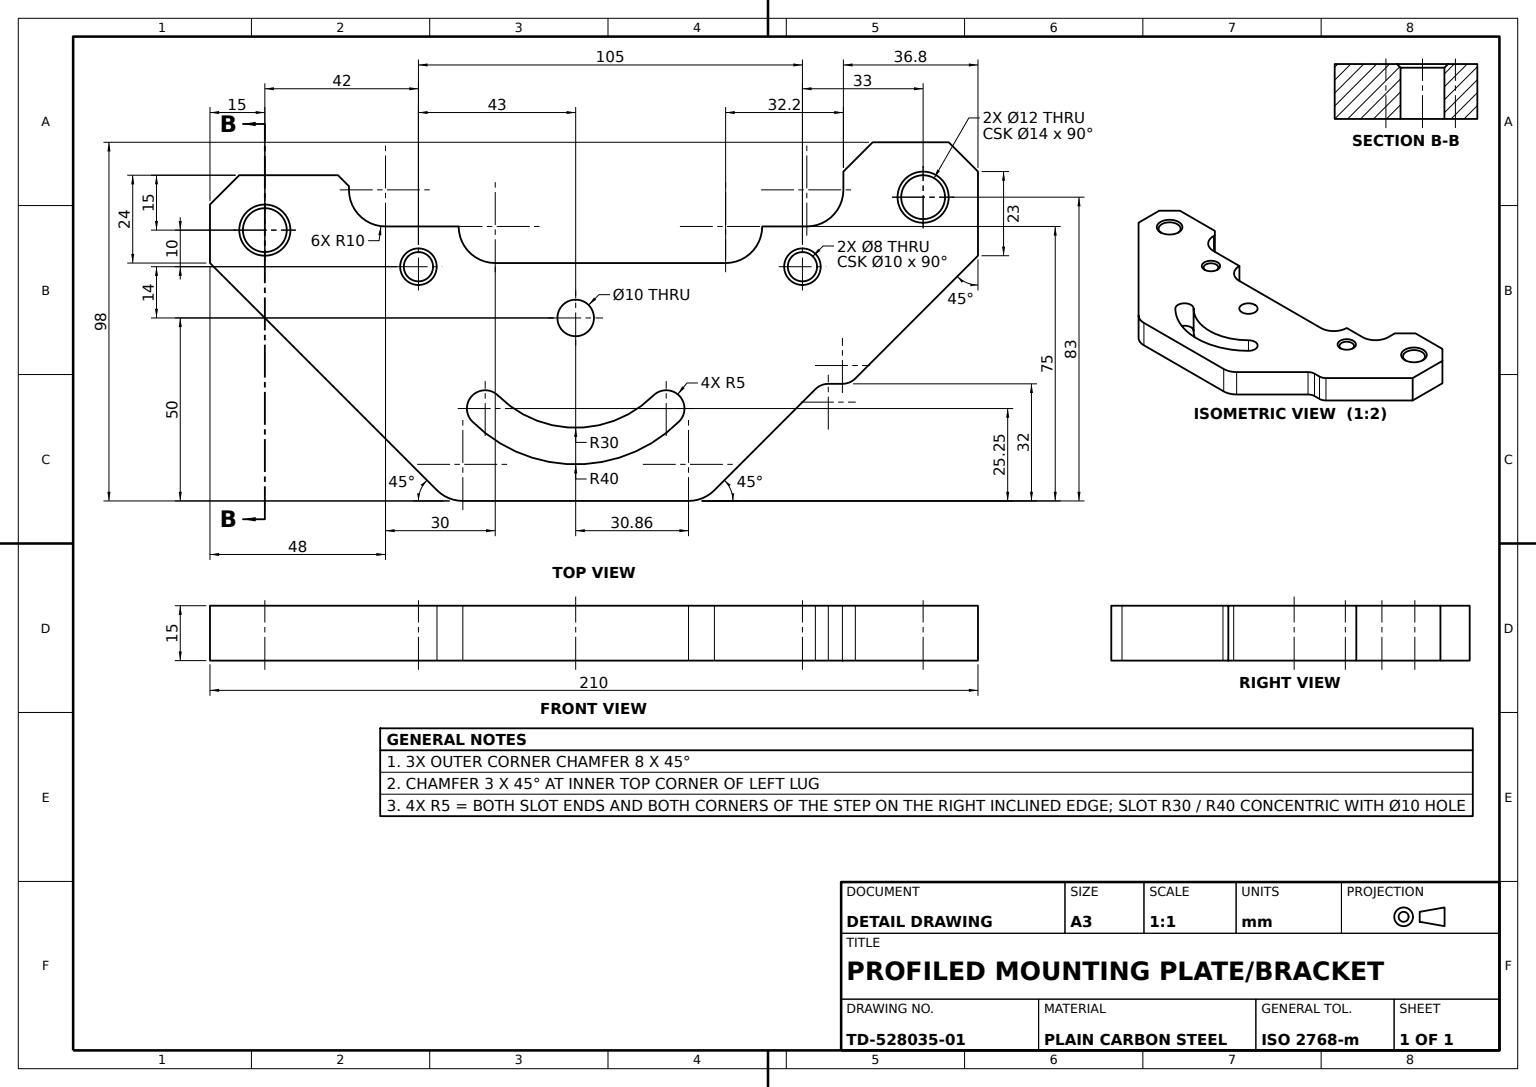
ISO-10303-21;
HEADER;
FILE_DESCRIPTION((''),'2;1');
FILE_NAME('','',(''),(''),'','','');
FILE_SCHEMA(('AUTOMOTIVE_DESIGN'));
ENDSEC;
DATA;
#1=APPLICATION_CONTEXT('');
#2=PRODUCT_CONTEXT('',#1,'mechanical');
#3=PRODUCT('','','',(#2));
#4=PRODUCT_DEFINITION_FORMATION('','',#3);
#5=PRODUCT_DEFINITION_CONTEXT('',#1,'design');
#6=PRODUCT_DEFINITION('','',#4,#5);
#7=PRODUCT_DEFINITION_SHAPE('','',#6);
#8=(LENGTH_UNIT()NAMED_UNIT(*)SI_UNIT(.MILLI.,.METRE.));
#9=(NAMED_UNIT(*)PLANE_ANGLE_UNIT()SI_UNIT($,.RADIAN.));
#10=(NAMED_UNIT(*)SI_UNIT($,.STERADIAN.)SOLID_ANGLE_UNIT());
#11=UNCERTAINTY_MEASURE_WITH_UNIT(LENGTH_MEASURE(1.E-05),#8,'distance_accuracy_value','');
#12=(GEOMETRIC_REPRESENTATION_CONTEXT(3)GLOBAL_UNCERTAINTY_ASSIGNED_CONTEXT((#11))GLOBAL_UNIT_ASSIGNED_CONTEXT((#8,#9,#10))REPRESENTATION_CONTEXT('',''));
#13=CARTESIAN_POINT('',(102.,15.,-48.));
#14=VERTEX_POINT('',#13);
#15=CARTESIAN_POINT('',(102.,0.,-48.));
#16=VERTEX_POINT('',#15);
#17=DIRECTION('',(0.,-1.,0.));
#18=VECTOR('',#17,1000.);
#19=LINE('',#13,#18);
#20=EDGE_CURVE('',#14,#16,#19,.T.);
#21=ORIENTED_EDGE('',*,*,#20,.F.);
#22=CARTESIAN_POINT('',(110.,15.,-40.));
#23=VERTEX_POINT('',#22);
#24=CARTESIAN_POINT('',(75.,15.,-75.));
#25=DIRECTION('',(-0.707106781,0.,-0.707106781));
#26=VECTOR('',#25,1000.);
#27=LINE('',#24,#26);
#28=EDGE_CURVE('',#23,#14,#27,.T.);
#29=ORIENTED_EDGE('',*,*,#28,.F.);
#30=CARTESIAN_POINT('',(110.,0.,-40.));
#31=VERTEX_POINT('',#30);
#32=DIRECTION('',(0.,1.,0.));
#33=VECTOR('',#32,1000.);
#34=LINE('',#22,#33);
#35=EDGE_CURVE('',#31,#23,#34,.T.);
#36=ORIENTED_EDGE('',*,*,#35,.F.);
#37=DIRECTION('',(0.707106781,0.,0.707106781));
#38=VECTOR('',#37,1000.);
#39=LINE('',#15,#38);
#40=EDGE_CURVE('',#16,#31,#39,.T.);
#41=ORIENTED_EDGE('',*,*,#40,.F.);
#42=EDGE_LOOP('',(#21,#29,#36,#41));
#43=FACE_OUTER_BOUND('',#42,.T.);
#44=DIRECTION('',(-0.707106781,0.,0.707106781));
#45=AXIS2_PLACEMENT_3D('',#13,#44,#17);
#46=PLANE('',#45);
#47=ADVANCED_FACE('',(#43),#46,.F.);
#48=CARTESIAN_POINT('',(-92.,0.,-39.));
#49=VERTEX_POINT('',#48);
#50=CARTESIAN_POINT('',(-65.,0.,-39.));
#51=VERTEX_POINT('',#50);
#52=CARTESIAN_POINT('',(0.,0.,-39.));
#53=DIRECTION('',(1.,0.,0.));
#54=VECTOR('',#53,1000.);
#55=LINE('',#52,#54);
#56=EDGE_CURVE('',#49,#51,#55,.T.);
#57=ORIENTED_EDGE('',*,*,#56,.F.);
#58=CARTESIAN_POINT('',(-92.,15.,-39.));
#59=VERTEX_POINT('',#58);
#60=LINE('',#58,#33);
#61=EDGE_CURVE('',#49,#59,#60,.T.);
#62=ORIENTED_EDGE('',*,*,#61,.T.);
#63=CARTESIAN_POINT('',(-65.,15.,-39.));
#64=VERTEX_POINT('',#63);
#65=CARTESIAN_POINT('',(0.,15.,-39.));
#66=LINE('',#65,#54);
#67=EDGE_CURVE('',#59,#64,#66,.T.);
#68=ORIENTED_EDGE('',*,*,#67,.T.);
#69=LINE('',#63,#18);
#70=EDGE_CURVE('',#64,#51,#69,.T.);
#71=ORIENTED_EDGE('',*,*,#70,.T.);
#72=EDGE_LOOP('',(#57,#62,#68,#71));
#73=FACE_OUTER_BOUND('',#72,.T.);
#74=DIRECTION('',(0.,0.,-1.));
#75=DIRECTION('',(-1.,0.,0.));
#76=AXIS2_PLACEMENT_3D('',#65,#74,#75);
#77=PLANE('',#76);
#78=ADVANCED_FACE('',(#73),#77,.T.);
#79=CARTESIAN_POINT('',(95.,14.,-39.));
#80=VERTEX_POINT('',#79);
#81=CARTESIAN_POINT('',(95.,14.,-27.));
#82=VERTEX_POINT('',#81);
#83=CARTESIAN_POINT('',(95.,14.,-33.));
#84=DIRECTION('',(0.,0.,1.));
#85=AXIS2_PLACEMENT_3D('',#83,#32,#84);
#86=CIRCLE('',#85,6.);
#87=EDGE_CURVE('',#80,#82,#86,.T.);
#88=ORIENTED_EDGE('',*,*,#87,.F.);
#89=CARTESIAN_POINT('',(95.,15.,-40.));
#90=VERTEX_POINT('',#89);
#91=DIRECTION('',(0.,0.707106781,-0.707106781));
#92=VECTOR('',#91,1000.);
#93=LINE('',#79,#92);
#94=EDGE_CURVE('',#80,#90,#93,.T.);
#95=ORIENTED_EDGE('',*,*,#94,.T.);
#96=CARTESIAN_POINT('',(95.,15.,-26.));
#97=VERTEX_POINT('',#96);
#98=CARTESIAN_POINT('',(95.,15.,-33.));
#99=AXIS2_PLACEMENT_3D('',#98,#17,#84);
#100=CIRCLE('',#99,7.);
#101=EDGE_CURVE('',#97,#90,#100,.T.);
#102=ORIENTED_EDGE('',*,*,#101,.F.);
#103=DIRECTION('',(0.,0.707106781,0.707106781));
#104=VECTOR('',#103,1000.);
#105=LINE('',#81,#104);
#106=EDGE_CURVE('',#82,#97,#105,.T.);
#107=ORIENTED_EDGE('',*,*,#106,.F.);
#108=EDGE_LOOP('',(#88,#95,#102,#107));
#109=FACE_OUTER_BOUND('',#108,.T.);
#110=CONICAL_SURFACE('',#85,6.,0.785398163);
#111=ADVANCED_FACE('',(#109),#110,.F.);
#112=CARTESIAN_POINT('',(-32.,15.,-25.));
#113=VERTEX_POINT('',#112);
#114=CARTESIAN_POINT('',(-32.,0.,-25.));
#115=VERTEX_POINT('',#114);
#116=LINE('',#112,#18);
#117=EDGE_CURVE('',#113,#115,#116,.T.);
#118=ORIENTED_EDGE('',*,*,#117,.F.);
#119=CARTESIAN_POINT('',(-22.,15.,-15.));
#120=VERTEX_POINT('',#119);
#121=CARTESIAN_POINT('',(-22.,15.,-25.));
#122=AXIS2_PLACEMENT_3D('',#121,#17,#84);
#123=CIRCLE('',#122,10.);
#124=EDGE_CURVE('',#120,#113,#123,.T.);
#125=ORIENTED_EDGE('',*,*,#124,.F.);
#126=CARTESIAN_POINT('',(-22.,0.,-15.));
#127=VERTEX_POINT('',#126);
#128=LINE('',#119,#33);
#129=EDGE_CURVE('',#127,#120,#128,.T.);
#130=ORIENTED_EDGE('',*,*,#129,.F.);
#131=CARTESIAN_POINT('',(-22.,0.,-25.));
#132=AXIS2_PLACEMENT_3D('',#131,#32,#84);
#133=CIRCLE('',#132,10.);
#134=EDGE_CURVE('',#115,#127,#133,.T.);
#135=ORIENTED_EDGE('',*,*,#134,.F.);
#136=EDGE_LOOP('',(#118,#125,#130,#135));
#137=FACE_OUTER_BOUND('',#136,.T.);
#138=AXIS2_PLACEMENT_3D('',#121,#32,#84);
#139=CYLINDRICAL_SURFACE('',#138,10.);
#140=ADVANCED_FACE('',(#137),#139,.F.);
#141=CARTESIAN_POINT('',(37.928932,15.,47.071068));
#142=VERTEX_POINT('',#141);
#143=CARTESIAN_POINT('',(37.928932,0.,47.071068));
#144=VERTEX_POINT('',#143);
#145=LINE('',#141,#18);
#146=EDGE_CURVE('',#142,#144,#145,.T.);
#147=ORIENTED_EDGE('',*,*,#146,.F.);
#148=CARTESIAN_POINT('',(30.857864,15.,50.));
#149=VERTEX_POINT('',#148);
#150=CARTESIAN_POINT('',(30.857864,15.,40.));
#151=AXIS2_PLACEMENT_3D('',#150,#32,#84);
#152=CIRCLE('',#151,10.);
#153=EDGE_CURVE('',#149,#142,#152,.T.);
#154=ORIENTED_EDGE('',*,*,#153,.F.);
#155=CARTESIAN_POINT('',(30.857864,0.,50.));
#156=VERTEX_POINT('',#155);
#157=LINE('',#148,#33);
#158=EDGE_CURVE('',#156,#149,#157,.T.);
#159=ORIENTED_EDGE('',*,*,#158,.F.);
#160=CARTESIAN_POINT('',(30.857864,0.,40.));
#161=AXIS2_PLACEMENT_3D('',#160,#17,#84);
#162=CIRCLE('',#161,10.);
#163=EDGE_CURVE('',#144,#156,#162,.T.);
#164=ORIENTED_EDGE('',*,*,#163,.F.);
#165=EDGE_LOOP('',(#147,#154,#159,#164));
#166=FACE_OUTER_BOUND('',#165,.T.);
#167=AXIS2_PLACEMENT_3D('',#150,#17,#74);
#168=CYLINDRICAL_SURFACE('',#167,10.);
#169=ADVANCED_FACE('',(#166),#168,.T.);
#170=CARTESIAN_POINT('',(28.284271,0.,28.284271));
#171=VERTEX_POINT('',#170);
#172=CARTESIAN_POINT('',(24.748737,0.,19.748737));
#173=VERTEX_POINT('',#172);
#174=CARTESIAN_POINT('',(24.748737,0.,24.748737));
#175=AXIS2_PLACEMENT_3D('',#174,#32,#84);
#176=CIRCLE('',#175,5.);
#177=EDGE_CURVE('',#171,#173,#176,.T.);
#178=ORIENTED_EDGE('',*,*,#177,.F.);
#179=CARTESIAN_POINT('',(28.284271,15.,28.284271));
#180=VERTEX_POINT('',#179);
#181=LINE('',#179,#18);
#182=EDGE_CURVE('',#180,#171,#181,.T.);
#183=ORIENTED_EDGE('',*,*,#182,.F.);
#184=CARTESIAN_POINT('',(24.748737,15.,19.748737));
#185=VERTEX_POINT('',#184);
#186=CARTESIAN_POINT('',(24.748737,15.,24.748737));
#187=AXIS2_PLACEMENT_3D('',#186,#32,#84);
#188=CIRCLE('',#187,5.);
#189=EDGE_CURVE('',#180,#185,#188,.T.);
#190=ORIENTED_EDGE('',*,*,#189,.T.);
#191=LINE('',#184,#18);
#192=EDGE_CURVE('',#185,#173,#191,.T.);
#193=ORIENTED_EDGE('',*,*,#192,.T.);
#194=EDGE_LOOP('',(#178,#183,#190,#193));
#195=FACE_OUTER_BOUND('',#194,.T.);
#196=AXIS2_PLACEMENT_3D('',#186,#17,#74);
#197=CYLINDRICAL_SURFACE('',#196,5.);
#198=ADVANCED_FACE('',(#195),#197,.F.);
#199=CARTESIAN_POINT('',(110.,15.,-17.));
#200=VERTEX_POINT('',#199);
#201=CARTESIAN_POINT('',(110.,0.,-17.));
#202=VERTEX_POINT('',#201);
#203=LINE('',#199,#18);
#204=EDGE_CURVE('',#200,#202,#203,.T.);
#205=ORIENTED_EDGE('',*,*,#204,.T.);
#206=CARTESIAN_POINT('',(110.,0.,0.));
#207=VECTOR('',#74,1000.);
#208=LINE('',#206,#207);
#209=EDGE_CURVE('',#202,#31,#208,.T.);
#210=ORIENTED_EDGE('',*,*,#209,.T.);
#211=ORIENTED_EDGE('',*,*,#35,.T.);
#212=CARTESIAN_POINT('',(110.,15.,0.));
#213=LINE('',#212,#207);
#214=EDGE_CURVE('',#200,#23,#213,.T.);
#215=ORIENTED_EDGE('',*,*,#214,.F.);
#216=EDGE_LOOP('',(#205,#210,#211,#215));
#217=FACE_OUTER_BOUND('',#216,.T.);
#218=AXIS2_PLACEMENT_3D('',#212,#75,#84);
#219=PLANE('',#218);
#220=ADVANCED_FACE('',(#217),#219,.F.);
#221=CARTESIAN_POINT('',(-62.,15.,-35.));
#222=VERTEX_POINT('',#221);
#223=CARTESIAN_POINT('',(-62.,0.,-35.));
#224=VERTEX_POINT('',#223);
#225=LINE('',#223,#18);
#226=EDGE_CURVE('',#222,#224,#225,.T.);
#227=ORIENTED_EDGE('',*,*,#226,.F.);
#228=CARTESIAN_POINT('',(-52.,15.,-25.));
#229=VERTEX_POINT('',#228);
#230=CARTESIAN_POINT('',(-52.,15.,-35.));
#231=AXIS2_PLACEMENT_3D('',#230,#17,#84);
#232=CIRCLE('',#231,10.);
#233=EDGE_CURVE('',#229,#222,#232,.T.);
#234=ORIENTED_EDGE('',*,*,#233,.F.);
#235=CARTESIAN_POINT('',(-52.,0.,-25.));
#236=VERTEX_POINT('',#235);
#237=LINE('',#228,#33);
#238=EDGE_CURVE('',#236,#229,#237,.T.);
#239=ORIENTED_EDGE('',*,*,#238,.F.);
#240=CARTESIAN_POINT('',(-52.,0.,-35.));
#241=AXIS2_PLACEMENT_3D('',#240,#32,#84);
#242=CIRCLE('',#241,10.);
#243=EDGE_CURVE('',#224,#236,#242,.T.);
#244=ORIENTED_EDGE('',*,*,#243,.F.);
#245=EDGE_LOOP('',(#227,#234,#239,#244));
#246=FACE_OUTER_BOUND('',#245,.T.);
#247=AXIS2_PLACEMENT_3D('',#230,#32,#84);
#248=CYLINDRICAL_SURFACE('',#247,10.);
#249=ADVANCED_FACE('',(#246),#248,.F.);
#250=CARTESIAN_POINT('',(-43.,14.,-10.));
#251=VERTEX_POINT('',#250);
#252=CARTESIAN_POINT('',(-43.,14.,-18.));
#253=VERTEX_POINT('',#252);
#254=CARTESIAN_POINT('',(-43.,14.,-14.));
#255=AXIS2_PLACEMENT_3D('',#254,#32,#84);
#256=CIRCLE('',#255,4.);
#257=EDGE_CURVE('',#251,#253,#256,.T.);
#258=ORIENTED_EDGE('',*,*,#257,.F.);
#259=CARTESIAN_POINT('',(-43.,15.,-9.));
#260=VERTEX_POINT('',#259);
#261=LINE('',#250,#104);
#262=EDGE_CURVE('',#251,#260,#261,.T.);
#263=ORIENTED_EDGE('',*,*,#262,.T.);
#264=CARTESIAN_POINT('',(-43.,15.,-19.));
#265=VERTEX_POINT('',#264);
#266=CARTESIAN_POINT('',(-43.,15.,-14.));
#267=AXIS2_PLACEMENT_3D('',#266,#17,#84);
#268=CIRCLE('',#267,5.);
#269=EDGE_CURVE('',#265,#260,#268,.T.);
#270=ORIENTED_EDGE('',*,*,#269,.F.);
#271=LINE('',#252,#92);
#272=EDGE_CURVE('',#253,#265,#271,.T.);
#273=ORIENTED_EDGE('',*,*,#272,.F.);
#274=EDGE_LOOP('',(#258,#263,#270,#273));
#275=FACE_OUTER_BOUND('',#274,.T.);
#276=CONICAL_SURFACE('',#255,4.,0.785398163);
#277=ADVANCED_FACE('',(#275),#276,.F.);
#278=CARTESIAN_POINT('',(-28.284271,15.,28.284271));
#279=VERTEX_POINT('',#278);
#280=CARTESIAN_POINT('',(0.,15.,0.));
#281=AXIS2_PLACEMENT_3D('',#280,#32,#84);
#282=CIRCLE('',#281,40.);
#283=EDGE_CURVE('',#279,#180,#282,.T.);
#284=ORIENTED_EDGE('',*,*,#283,.T.);
#285=ORIENTED_EDGE('',*,*,#182,.T.);
#286=CARTESIAN_POINT('',(-28.284271,0.,28.284271));
#287=VERTEX_POINT('',#286);
#288=CARTESIAN_POINT('',(0.,0.,0.));
#289=AXIS2_PLACEMENT_3D('',#288,#32,#84);
#290=CIRCLE('',#289,40.);
#291=EDGE_CURVE('',#287,#171,#290,.T.);
#292=ORIENTED_EDGE('',*,*,#291,.F.);
#293=LINE('',#278,#18);
#294=EDGE_CURVE('',#279,#287,#293,.T.);
#295=ORIENTED_EDGE('',*,*,#294,.F.);
#296=EDGE_LOOP('',(#284,#285,#292,#295));
#297=FACE_OUTER_BOUND('',#296,.T.);
#298=AXIS2_PLACEMENT_3D('',#280,#17,#74);
#299=CYLINDRICAL_SURFACE('',#298,40.);
#300=ADVANCED_FACE('',(#297),#299,.F.);
#301=CARTESIAN_POINT('',(-30.857864,15.,50.));
#302=VERTEX_POINT('',#301);
#303=CARTESIAN_POINT('',(-30.857864,0.,50.));
#304=VERTEX_POINT('',#303);
#305=LINE('',#303,#18);
#306=EDGE_CURVE('',#302,#304,#305,.T.);
#307=ORIENTED_EDGE('',*,*,#306,.F.);
#308=CARTESIAN_POINT('',(-37.928932,15.,47.071068));
#309=VERTEX_POINT('',#308);
#310=CARTESIAN_POINT('',(-30.857864,15.,40.));
#311=AXIS2_PLACEMENT_3D('',#310,#32,#84);
#312=CIRCLE('',#311,10.);
#313=EDGE_CURVE('',#309,#302,#312,.T.);
#314=ORIENTED_EDGE('',*,*,#313,.F.);
#315=CARTESIAN_POINT('',(-37.928932,0.,47.071068));
#316=VERTEX_POINT('',#315);
#317=LINE('',#308,#33);
#318=EDGE_CURVE('',#316,#309,#317,.T.);
#319=ORIENTED_EDGE('',*,*,#318,.F.);
#320=CARTESIAN_POINT('',(-30.857864,0.,40.));
#321=AXIS2_PLACEMENT_3D('',#320,#17,#84);
#322=CIRCLE('',#321,10.);
#323=EDGE_CURVE('',#304,#316,#322,.T.);
#324=ORIENTED_EDGE('',*,*,#323,.F.);
#325=EDGE_LOOP('',(#307,#314,#319,#324));
#326=FACE_OUTER_BOUND('',#325,.T.);
#327=CYLINDRICAL_SURFACE('',#311,10.);
#328=ADVANCED_FACE('',(#326),#327,.T.);
#329=CARTESIAN_POINT('',(41.,15.,-15.));
#330=VERTEX_POINT('',#329);
#331=CARTESIAN_POINT('',(41.,0.,-15.));
#332=VERTEX_POINT('',#331);
#333=LINE('',#329,#18);
#334=EDGE_CURVE('',#330,#332,#333,.T.);
#335=ORIENTED_EDGE('',*,*,#334,.F.);
#336=CARTESIAN_POINT('',(51.,15.,-25.));
#337=VERTEX_POINT('',#336);
#338=CARTESIAN_POINT('',(41.,15.,-25.));
#339=AXIS2_PLACEMENT_3D('',#338,#17,#84);
#340=CIRCLE('',#339,10.);
#341=EDGE_CURVE('',#337,#330,#340,.T.);
#342=ORIENTED_EDGE('',*,*,#341,.F.);
#343=CARTESIAN_POINT('',(51.,0.,-25.));
#344=VERTEX_POINT('',#343);
#345=LINE('',#336,#18);
#346=EDGE_CURVE('',#337,#344,#345,.T.);
#347=ORIENTED_EDGE('',*,*,#346,.T.);
#348=CARTESIAN_POINT('',(41.,0.,-25.));
#349=AXIS2_PLACEMENT_3D('',#348,#32,#84);
#350=CIRCLE('',#349,10.);
#351=EDGE_CURVE('',#332,#344,#350,.T.);
#352=ORIENTED_EDGE('',*,*,#351,.F.);
#353=EDGE_LOOP('',(#335,#342,#347,#352));
#354=FACE_OUTER_BOUND('',#353,.T.);
#355=AXIS2_PLACEMENT_3D('',#338,#17,#74);
#356=CYLINDRICAL_SURFACE('',#355,10.);
#357=ADVANCED_FACE('',(#354),#356,.F.);
#358=CARTESIAN_POINT('',(62.,14.,-18.));
#359=VERTEX_POINT('',#358);
#360=CARTESIAN_POINT('',(62.,15.,-19.));
#361=VERTEX_POINT('',#360);
#362=LINE('',#358,#92);
#363=EDGE_CURVE('',#359,#361,#362,.T.);
#364=ORIENTED_EDGE('',*,*,#363,.T.);
#365=CARTESIAN_POINT('',(62.,15.,-9.));
#366=VERTEX_POINT('',#365);
#367=CARTESIAN_POINT('',(62.,15.,-14.));
#368=AXIS2_PLACEMENT_3D('',#367,#17,#84);
#369=CIRCLE('',#368,5.);
#370=EDGE_CURVE('',#366,#361,#369,.T.);
#371=ORIENTED_EDGE('',*,*,#370,.F.);
#372=CARTESIAN_POINT('',(62.,14.,-10.));
#373=VERTEX_POINT('',#372);
#374=LINE('',#372,#104);
#375=EDGE_CURVE('',#373,#366,#374,.T.);
#376=ORIENTED_EDGE('',*,*,#375,.F.);
#377=CARTESIAN_POINT('',(62.,14.,-14.));
#378=AXIS2_PLACEMENT_3D('',#377,#32,#84);
#379=CIRCLE('',#378,4.);
#380=EDGE_CURVE('',#359,#373,#379,.T.);
#381=ORIENTED_EDGE('',*,*,#380,.F.);
#382=EDGE_LOOP('',(#364,#371,#376,#381));
#383=FACE_OUTER_BOUND('',#382,.T.);
#384=CONICAL_SURFACE('',#378,4.,0.785398163);
#385=ADVANCED_FACE('',(#383),#384,.F.);
#386=CARTESIAN_POINT('',(-43.,0.,-10.));
#387=VERTEX_POINT('',#386);
#388=CARTESIAN_POINT('',(-43.,15.,-10.));
#389=LINE('',#388,#33);
#390=EDGE_CURVE('',#387,#251,#389,.T.);
#391=ORIENTED_EDGE('',*,*,#390,.T.);
#392=ORIENTED_EDGE('',*,*,#257,.T.);
#393=CARTESIAN_POINT('',(-43.,0.,-18.));
#394=VERTEX_POINT('',#393);
#395=CARTESIAN_POINT('',(-43.,15.,-18.));
#396=LINE('',#395,#33);
#397=EDGE_CURVE('',#394,#253,#396,.T.);
#398=ORIENTED_EDGE('',*,*,#397,.F.);
#399=CARTESIAN_POINT('',(-43.,0.,-14.));
#400=AXIS2_PLACEMENT_3D('',#399,#32,#84);
#401=CIRCLE('',#400,4.);
#402=EDGE_CURVE('',#387,#394,#401,.T.);
#403=ORIENTED_EDGE('',*,*,#402,.F.);
#404=EDGE_LOOP('',(#391,#392,#398,#403));
#405=FACE_OUTER_BOUND('',#404,.T.);
#406=AXIS2_PLACEMENT_3D('',#266,#32,#84);
#407=CYLINDRICAL_SURFACE('',#406,4.);
#408=ADVANCED_FACE('',(#405),#407,.F.);
#409=ORIENTED_EDGE('',*,*,#346,.F.);
#410=CARTESIAN_POINT('',(63.200292,15.,-25.));
#411=VERTEX_POINT('',#410);
#412=CARTESIAN_POINT('',(0.,15.,-25.));
#413=VECTOR('',#75,1000.);
#414=LINE('',#412,#413);
#415=EDGE_CURVE('',#411,#337,#414,.T.);
#416=ORIENTED_EDGE('',*,*,#415,.F.);
#417=CARTESIAN_POINT('',(63.200292,0.,-25.));
#418=VERTEX_POINT('',#417);
#419=LINE('',#417,#18);
#420=EDGE_CURVE('',#411,#418,#419,.T.);
#421=ORIENTED_EDGE('',*,*,#420,.T.);
#422=CARTESIAN_POINT('',(0.,0.,-25.));
#423=LINE('',#422,#413);
#424=EDGE_CURVE('',#418,#344,#423,.T.);
#425=ORIENTED_EDGE('',*,*,#424,.T.);
#426=EDGE_LOOP('',(#409,#416,#421,#425));
#427=FACE_OUTER_BOUND('',#426,.T.);
#428=AXIS2_PLACEMENT_3D('',#412,#84,#53);
#429=PLANE('',#428);
#430=ADVANCED_FACE('',(#427),#429,.F.);
#431=ORIENTED_EDGE('',*,*,#375,.T.);
#432=EDGE_CURVE('',#361,#366,#369,.T.);
#433=ORIENTED_EDGE('',*,*,#432,.F.);
#434=ORIENTED_EDGE('',*,*,#363,.F.);
#435=EDGE_CURVE('',#373,#359,#379,.T.);
#436=ORIENTED_EDGE('',*,*,#435,.F.);
#437=EDGE_LOOP('',(#431,#433,#434,#436));
#438=FACE_OUTER_BOUND('',#437,.T.);
#439=ADVANCED_FACE('',(#438),#384,.F.);
#440=CARTESIAN_POINT('',(-24.748737,0.,19.748737));
#441=VERTEX_POINT('',#440);
#442=CARTESIAN_POINT('',(-24.748737,0.,24.748737));
#443=AXIS2_PLACEMENT_3D('',#442,#32,#84);
#444=CIRCLE('',#443,5.);
#445=EDGE_CURVE('',#441,#287,#444,.T.);
#446=ORIENTED_EDGE('',*,*,#445,.F.);
#447=CARTESIAN_POINT('',(-24.748737,15.,19.748737));
#448=VERTEX_POINT('',#447);
#449=LINE('',#447,#18);
#450=EDGE_CURVE('',#448,#441,#449,.T.);
#451=ORIENTED_EDGE('',*,*,#450,.F.);
#452=CARTESIAN_POINT('',(-24.748737,15.,24.748737));
#453=AXIS2_PLACEMENT_3D('',#452,#32,#84);
#454=CIRCLE('',#453,5.);
#455=EDGE_CURVE('',#448,#279,#454,.T.);
#456=ORIENTED_EDGE('',*,*,#455,.T.);
#457=ORIENTED_EDGE('',*,*,#294,.T.);
#458=EDGE_LOOP('',(#446,#451,#456,#457));
#459=FACE_OUTER_BOUND('',#458,.T.);
#460=AXIS2_PLACEMENT_3D('',#452,#17,#74);
#461=CYLINDRICAL_SURFACE('',#460,5.);
#462=ADVANCED_FACE('',(#459),#461,.F.);
#463=CARTESIAN_POINT('',(-62.,0.,-36.));
#464=VERTEX_POINT('',#463);
#465=CARTESIAN_POINT('',(-62.,0.,0.));
#466=VECTOR('',#84,1000.);
#467=LINE('',#465,#466);
#468=EDGE_CURVE('',#464,#224,#467,.T.);
#469=ORIENTED_EDGE('',*,*,#468,.F.);
#470=CARTESIAN_POINT('',(-62.,15.,-36.));
#471=VERTEX_POINT('',#470);
#472=LINE('',#470,#33);
#473=EDGE_CURVE('',#464,#471,#472,.T.);
#474=ORIENTED_EDGE('',*,*,#473,.T.);
#475=CARTESIAN_POINT('',(-62.,15.,0.));
#476=LINE('',#475,#466);
#477=EDGE_CURVE('',#471,#222,#476,.T.);
#478=ORIENTED_EDGE('',*,*,#477,.T.);
#479=ORIENTED_EDGE('',*,*,#226,.T.);
#480=EDGE_LOOP('',(#469,#474,#478,#479));
#481=FACE_OUTER_BOUND('',#480,.T.);
#482=AXIS2_PLACEMENT_3D('',#475,#53,#74);
#483=PLANE('',#482);
#484=ADVANCED_FACE('',(#481),#483,.T.);
#485=CARTESIAN_POINT('',(65.535534,15.,19.464466));
#486=VERTEX_POINT('',#485);
#487=CARTESIAN_POINT('',(42.5,15.,42.5));
#488=DIRECTION('',(0.707106781,0.,-0.707106781));
#489=VECTOR('',#488,1000.);
#490=LINE('',#487,#489);
#491=EDGE_CURVE('',#142,#486,#490,.T.);
#492=ORIENTED_EDGE('',*,*,#491,.T.);
#493=CARTESIAN_POINT('',(69.071068,15.,18.));
#494=VERTEX_POINT('',#493);
#495=CARTESIAN_POINT('',(69.071068,15.,23.));
#496=AXIS2_PLACEMENT_3D('',#495,#17,#84);
#497=CIRCLE('',#496,5.);
#498=EDGE_CURVE('',#486,#494,#497,.T.);
#499=ORIENTED_EDGE('',*,*,#498,.T.);
#500=CARTESIAN_POINT('',(72.928932,15.,18.));
#501=VERTEX_POINT('',#500);
#502=CARTESIAN_POINT('',(0.,15.,18.));
#503=LINE('',#502,#413);
#504=EDGE_CURVE('',#501,#494,#503,.T.);
#505=ORIENTED_EDGE('',*,*,#504,.F.);
#506=CARTESIAN_POINT('',(76.464466,15.,16.535534));
#507=VERTEX_POINT('',#506);
#508=CARTESIAN_POINT('',(72.928932,15.,13.));
#509=AXIS2_PLACEMENT_3D('',#508,#32,#84);
#510=CIRCLE('',#509,5.);
#511=EDGE_CURVE('',#501,#507,#510,.T.);
#512=ORIENTED_EDGE('',*,*,#511,.T.);
#513=CARTESIAN_POINT('',(46.5,15.,46.5));
#514=VECTOR('',#44,1000.);
#515=LINE('',#513,#514);
#516=EDGE_CURVE('',#200,#507,#515,.T.);
#517=ORIENTED_EDGE('',*,*,#516,.F.);
#518=ORIENTED_EDGE('',*,*,#214,.T.);
#519=ORIENTED_EDGE('',*,*,#28,.T.);
#520=CARTESIAN_POINT('',(81.200292,15.,-48.));
#521=VERTEX_POINT('',#520);
#522=CARTESIAN_POINT('',(0.,15.,-48.));
#523=LINE('',#522,#413);
#524=EDGE_CURVE('',#14,#521,#523,.T.);
#525=ORIENTED_EDGE('',*,*,#524,.T.);
#526=CARTESIAN_POINT('',(73.200292,15.,-40.));
#527=VERTEX_POINT('',#526);
#528=CARTESIAN_POINT('',(16.600146,15.,16.600146));
#529=LINE('',#528,#514);
#530=EDGE_CURVE('',#521,#527,#529,.T.);
#531=ORIENTED_EDGE('',*,*,#530,.T.);
#532=CARTESIAN_POINT('',(73.200292,15.,-35.));
#533=VERTEX_POINT('',#532);
#534=CARTESIAN_POINT('',(73.200292,15.,0.));
#535=LINE('',#534,#466);
#536=EDGE_CURVE('',#527,#533,#535,.T.);
#537=ORIENTED_EDGE('',*,*,#536,.T.);
#538=CARTESIAN_POINT('',(63.200292,15.,-35.));
#539=AXIS2_PLACEMENT_3D('',#538,#17,#84);
#540=CIRCLE('',#539,10.);
#541=EDGE_CURVE('',#533,#411,#540,.T.);
#542=ORIENTED_EDGE('',*,*,#541,.T.);
#543=ORIENTED_EDGE('',*,*,#415,.T.);
#544=ORIENTED_EDGE('',*,*,#341,.T.);
#545=CARTESIAN_POINT('',(0.,15.,-15.));
#546=LINE('',#545,#54);
#547=EDGE_CURVE('',#120,#330,#546,.T.);
#548=ORIENTED_EDGE('',*,*,#547,.F.);
#549=ORIENTED_EDGE('',*,*,#124,.T.);
#550=LINE('',#412,#54);
#551=EDGE_CURVE('',#229,#113,#550,.T.);
#552=ORIENTED_EDGE('',*,*,#551,.F.);
#553=ORIENTED_EDGE('',*,*,#233,.T.);
#554=ORIENTED_EDGE('',*,*,#477,.F.);
#555=CARTESIAN_POINT('',(-13.,15.,13.));
#556=LINE('',#555,#26);
#557=EDGE_CURVE('',#471,#64,#556,.T.);
#558=ORIENTED_EDGE('',*,*,#557,.T.);
#559=ORIENTED_EDGE('',*,*,#67,.F.);
#560=CARTESIAN_POINT('',(-100.,15.,-31.));
#561=VERTEX_POINT('',#560);
#562=CARTESIAN_POINT('',(-65.5,15.,-65.5));
#563=LINE('',#562,#514);
#564=EDGE_CURVE('',#59,#561,#563,.T.);
#565=ORIENTED_EDGE('',*,*,#564,.T.);
#566=CARTESIAN_POINT('',(-100.,15.,-15.));
#567=VERTEX_POINT('',#566);
#568=CARTESIAN_POINT('',(-100.,15.,0.));
#569=LINE('',#568,#207);
#570=EDGE_CURVE('',#567,#561,#569,.T.);
#571=ORIENTED_EDGE('',*,*,#570,.F.);
#572=CARTESIAN_POINT('',(-42.5,15.,42.5));
#573=LINE('',#572,#26);
#574=EDGE_CURVE('',#309,#567,#573,.T.);
#575=ORIENTED_EDGE('',*,*,#574,.F.);
#576=ORIENTED_EDGE('',*,*,#313,.T.);
#577=CARTESIAN_POINT('',(0.,15.,50.));
#578=LINE('',#577,#54);
#579=EDGE_CURVE('',#302,#149,#578,.T.);
#580=ORIENTED_EDGE('',*,*,#579,.T.);
#581=ORIENTED_EDGE('',*,*,#153,.T.);
#582=EDGE_LOOP('',(#492,#499,#505,#512,#517,#518,#519,#525,#531,#537,#542,#543,#544,#548,#549,#552,#553,#554,#558,#559,#565,#571,#575,#576,#580,#581));
#583=FACE_OUTER_BOUND('',#582,.T.);
#584=EDGE_CURVE('',#90,#97,#100,.T.);
#585=ORIENTED_EDGE('',*,*,#584,.T.);
#586=ORIENTED_EDGE('',*,*,#101,.T.);
#587=EDGE_LOOP('',(#585,#586));
#588=FACE_BOUND('',#587,.T.);
#589=ORIENTED_EDGE('',*,*,#432,.T.);
#590=ORIENTED_EDGE('',*,*,#370,.T.);
#591=EDGE_LOOP('',(#589,#590));
#592=FACE_BOUND('',#591,.T.);
#593=EDGE_CURVE('',#260,#265,#268,.T.);
#594=ORIENTED_EDGE('',*,*,#593,.T.);
#595=ORIENTED_EDGE('',*,*,#269,.T.);
#596=EDGE_LOOP('',(#594,#595));
#597=FACE_BOUND('',#596,.T.);
#598=CARTESIAN_POINT('',(-85.,15.,-17.));
#599=VERTEX_POINT('',#598);
#600=CARTESIAN_POINT('',(-85.,15.,-31.));
#601=VERTEX_POINT('',#600);
#602=CARTESIAN_POINT('',(-85.,15.,-24.));
#603=AXIS2_PLACEMENT_3D('',#602,#17,#84);
#604=CIRCLE('',#603,7.);
#605=EDGE_CURVE('',#599,#601,#604,.T.);
#606=ORIENTED_EDGE('',*,*,#605,.T.);
#607=EDGE_CURVE('',#601,#599,#604,.T.);
#608=ORIENTED_EDGE('',*,*,#607,.T.);
#609=EDGE_LOOP('',(#606,#608));
#610=FACE_BOUND('',#609,.T.);
#611=ORIENTED_EDGE('',*,*,#189,.F.);
#612=ORIENTED_EDGE('',*,*,#283,.F.);
#613=ORIENTED_EDGE('',*,*,#455,.F.);
#614=CARTESIAN_POINT('',(-21.213203,15.,21.213203));
#615=VERTEX_POINT('',#614);
#616=EDGE_CURVE('',#615,#448,#454,.T.);
#617=ORIENTED_EDGE('',*,*,#616,.F.);
#618=CARTESIAN_POINT('',(21.213203,15.,21.213203));
#619=VERTEX_POINT('',#618);
#620=CIRCLE('',#281,30.);
#621=EDGE_CURVE('',#615,#619,#620,.T.);
#622=ORIENTED_EDGE('',*,*,#621,.T.);
#623=EDGE_CURVE('',#185,#619,#188,.T.);
#624=ORIENTED_EDGE('',*,*,#623,.F.);
#625=EDGE_LOOP('',(#611,#612,#613,#617,#622,#624));
#626=FACE_BOUND('',#625,.T.);
#627=CARTESIAN_POINT('',(0.,15.,-5.));
#628=VERTEX_POINT('',#627);
#629=CARTESIAN_POINT('',(0.,15.,5.));
#630=VERTEX_POINT('',#629);
#631=CIRCLE('',#281,5.);
#632=EDGE_CURVE('',#628,#630,#631,.T.);
#633=ORIENTED_EDGE('',*,*,#632,.F.);
#634=EDGE_CURVE('',#630,#628,#631,.T.);
#635=ORIENTED_EDGE('',*,*,#634,.F.);
#636=EDGE_LOOP('',(#633,#635));
#637=FACE_BOUND('',#636,.T.);
#638=PLANE('',#281);
#639=ADVANCED_FACE('',(#583,#588,#592,#597,#610,#626,#637),#638,.T.);
#640=ORIENTED_EDGE('',*,*,#94,.F.);
#641=EDGE_CURVE('',#82,#80,#86,.T.);
#642=ORIENTED_EDGE('',*,*,#641,.F.);
#643=ORIENTED_EDGE('',*,*,#106,.T.);
#644=ORIENTED_EDGE('',*,*,#584,.F.);
#645=EDGE_LOOP('',(#640,#642,#643,#644));
#646=FACE_OUTER_BOUND('',#645,.T.);
#647=ADVANCED_FACE('',(#646),#110,.F.);
#648=ORIENTED_EDGE('',*,*,#579,.F.);
#649=ORIENTED_EDGE('',*,*,#306,.T.);
#650=CARTESIAN_POINT('',(0.,0.,50.));
#651=LINE('',#650,#54);
#652=EDGE_CURVE('',#304,#156,#651,.T.);
#653=ORIENTED_EDGE('',*,*,#652,.T.);
#654=ORIENTED_EDGE('',*,*,#158,.T.);
#655=EDGE_LOOP('',(#648,#649,#653,#654));
#656=FACE_OUTER_BOUND('',#655,.T.);
#657=AXIS2_PLACEMENT_3D('',#577,#74,#75);
#658=PLANE('',#657);
#659=ADVANCED_FACE('',(#656),#658,.F.);
#660=CARTESIAN_POINT('',(95.,0.,-39.));
#661=VERTEX_POINT('',#660);
#662=CARTESIAN_POINT('',(95.,15.,-39.));
#663=LINE('',#662,#33);
#664=EDGE_CURVE('',#661,#80,#663,.T.);
#665=ORIENTED_EDGE('',*,*,#664,.T.);
#666=ORIENTED_EDGE('',*,*,#87,.T.);
#667=CARTESIAN_POINT('',(95.,0.,-27.));
#668=VERTEX_POINT('',#667);
#669=CARTESIAN_POINT('',(95.,15.,-27.));
#670=LINE('',#669,#33);
#671=EDGE_CURVE('',#668,#82,#670,.T.);
#672=ORIENTED_EDGE('',*,*,#671,.F.);
#673=CARTESIAN_POINT('',(95.,0.,-33.));
#674=AXIS2_PLACEMENT_3D('',#673,#32,#84);
#675=CIRCLE('',#674,6.);
#676=EDGE_CURVE('',#661,#668,#675,.T.);
#677=ORIENTED_EDGE('',*,*,#676,.F.);
#678=EDGE_LOOP('',(#665,#666,#672,#677));
#679=FACE_OUTER_BOUND('',#678,.T.);
#680=AXIS2_PLACEMENT_3D('',#98,#32,#84);
#681=CYLINDRICAL_SURFACE('',#680,6.);
#682=ADVANCED_FACE('',(#679),#681,.F.);
#683=CARTESIAN_POINT('',(-85.,0.,-30.));
#684=VERTEX_POINT('',#683);
#685=CARTESIAN_POINT('',(-85.,14.,-30.));
#686=VERTEX_POINT('',#685);
#687=CARTESIAN_POINT('',(-85.,15.,-30.));
#688=LINE('',#687,#33);
#689=EDGE_CURVE('',#684,#686,#688,.T.);
#690=ORIENTED_EDGE('',*,*,#689,.F.);
#691=CARTESIAN_POINT('',(-85.,0.,-18.));
#692=VERTEX_POINT('',#691);
#693=CARTESIAN_POINT('',(-85.,0.,-24.));
#694=AXIS2_PLACEMENT_3D('',#693,#32,#84);
#695=CIRCLE('',#694,6.);
#696=EDGE_CURVE('',#692,#684,#695,.T.);
#697=ORIENTED_EDGE('',*,*,#696,.F.);
#698=CARTESIAN_POINT('',(-85.,14.,-18.));
#699=VERTEX_POINT('',#698);
#700=CARTESIAN_POINT('',(-85.,15.,-18.));
#701=LINE('',#700,#33);
#702=EDGE_CURVE('',#692,#699,#701,.T.);
#703=ORIENTED_EDGE('',*,*,#702,.T.);
#704=CARTESIAN_POINT('',(-85.,14.,-24.));
#705=AXIS2_PLACEMENT_3D('',#704,#32,#84);
#706=CIRCLE('',#705,6.);
#707=EDGE_CURVE('',#699,#686,#706,.T.);
#708=ORIENTED_EDGE('',*,*,#707,.T.);
#709=EDGE_LOOP('',(#690,#697,#703,#708));
#710=FACE_OUTER_BOUND('',#709,.T.);
#711=AXIS2_PLACEMENT_3D('',#602,#32,#84);
#712=CYLINDRICAL_SURFACE('',#711,6.);
#713=ADVANCED_FACE('',(#710),#712,.F.);
#714=ORIENTED_EDGE('',*,*,#616,.T.);
#715=ORIENTED_EDGE('',*,*,#450,.T.);
#716=CARTESIAN_POINT('',(-21.213203,0.,21.213203));
#717=VERTEX_POINT('',#716);
#718=EDGE_CURVE('',#717,#441,#444,.T.);
#719=ORIENTED_EDGE('',*,*,#718,.F.);
#720=LINE('',#614,#18);
#721=EDGE_CURVE('',#615,#717,#720,.T.);
#722=ORIENTED_EDGE('',*,*,#721,.F.);
#723=EDGE_LOOP('',(#714,#715,#719,#722));
#724=FACE_OUTER_BOUND('',#723,.T.);
#725=ADVANCED_FACE('',(#724),#461,.F.);
#726=ORIENTED_EDGE('',*,*,#564,.F.);
#727=ORIENTED_EDGE('',*,*,#61,.F.);
#728=CARTESIAN_POINT('',(-100.,0.,-31.));
#729=VERTEX_POINT('',#728);
#730=LINE('',#728,#489);
#731=EDGE_CURVE('',#729,#49,#730,.T.);
#732=ORIENTED_EDGE('',*,*,#731,.F.);
#733=LINE('',#560,#18);
#734=EDGE_CURVE('',#561,#729,#733,.T.);
#735=ORIENTED_EDGE('',*,*,#734,.F.);
#736=EDGE_LOOP('',(#726,#727,#732,#735));
#737=FACE_OUTER_BOUND('',#736,.T.);
#738=AXIS2_PLACEMENT_3D('',#560,#37,#17);
#739=PLANE('',#738);
#740=ADVANCED_FACE('',(#737),#739,.F.);
#741=CARTESIAN_POINT('',(-100.,0.,-15.));
#742=VERTEX_POINT('',#741);
#743=LINE('',#566,#18);
#744=EDGE_CURVE('',#567,#742,#743,.T.);
#745=ORIENTED_EDGE('',*,*,#744,.T.);
#746=CARTESIAN_POINT('',(-42.5,0.,42.5));
#747=LINE('',#746,#26);
#748=EDGE_CURVE('',#316,#742,#747,.T.);
#749=ORIENTED_EDGE('',*,*,#748,.F.);
#750=ORIENTED_EDGE('',*,*,#318,.T.);
#751=ORIENTED_EDGE('',*,*,#574,.T.);
#752=EDGE_LOOP('',(#745,#749,#750,#751));
#753=FACE_OUTER_BOUND('',#752,.T.);
#754=AXIS2_PLACEMENT_3D('',#572,#44,#37);
#755=PLANE('',#754);
#756=ADVANCED_FACE('',(#753),#755,.T.);
#757=ORIENTED_EDGE('',*,*,#641,.T.);
#758=ORIENTED_EDGE('',*,*,#664,.F.);
#759=EDGE_CURVE('',#668,#661,#675,.T.);
#760=ORIENTED_EDGE('',*,*,#759,.F.);
#761=ORIENTED_EDGE('',*,*,#671,.T.);
#762=EDGE_LOOP('',(#757,#758,#760,#761));
#763=FACE_OUTER_BOUND('',#762,.T.);
#764=ADVANCED_FACE('',(#763),#681,.F.);
#765=CARTESIAN_POINT('',(69.071068,0.,18.));
#766=VERTEX_POINT('',#765);
#767=LINE('',#493,#18);
#768=EDGE_CURVE('',#494,#766,#767,.T.);
#769=ORIENTED_EDGE('',*,*,#768,.T.);
#770=CARTESIAN_POINT('',(72.928932,0.,18.));
#771=VERTEX_POINT('',#770);
#772=CARTESIAN_POINT('',(0.,0.,18.));
#773=LINE('',#772,#413);
#774=EDGE_CURVE('',#771,#766,#773,.T.);
#775=ORIENTED_EDGE('',*,*,#774,.F.);
#776=LINE('',#500,#33);
#777=EDGE_CURVE('',#771,#501,#776,.T.);
#778=ORIENTED_EDGE('',*,*,#777,.T.);
#779=ORIENTED_EDGE('',*,*,#504,.T.);
#780=EDGE_LOOP('',(#769,#775,#778,#779));
#781=FACE_OUTER_BOUND('',#780,.T.);
#782=AXIS2_PLACEMENT_3D('',#502,#84,#53);
#783=PLANE('',#782);
#784=ADVANCED_FACE('',(#781),#783,.T.);
#785=CARTESIAN_POINT('',(0.,0.,-5.));
#786=VERTEX_POINT('',#785);
#787=CARTESIAN_POINT('',(0.,0.,5.));
#788=VERTEX_POINT('',#787);
#789=CIRCLE('',#289,5.);
#790=EDGE_CURVE('',#786,#788,#789,.T.);
#791=ORIENTED_EDGE('',*,*,#790,.F.);
#792=LINE('',#627,#18);
#793=EDGE_CURVE('',#628,#786,#792,.T.);
#794=ORIENTED_EDGE('',*,*,#793,.F.);
#795=ORIENTED_EDGE('',*,*,#632,.T.);
#796=LINE('',#629,#18);
#797=EDGE_CURVE('',#630,#788,#796,.T.);
#798=ORIENTED_EDGE('',*,*,#797,.T.);
#799=EDGE_LOOP('',(#791,#794,#795,#798));
#800=FACE_OUTER_BOUND('',#799,.T.);
#801=CYLINDRICAL_SURFACE('',#298,5.);
#802=ADVANCED_FACE('',(#800),#801,.F.);
#803=LINE('',#685,#92);
#804=EDGE_CURVE('',#686,#601,#803,.T.);
#805=ORIENTED_EDGE('',*,*,#804,.F.);
#806=ORIENTED_EDGE('',*,*,#707,.F.);
#807=LINE('',#698,#104);
#808=EDGE_CURVE('',#699,#599,#807,.T.);
#809=ORIENTED_EDGE('',*,*,#808,.T.);
#810=ORIENTED_EDGE('',*,*,#607,.F.);
#811=EDGE_LOOP('',(#805,#806,#809,#810));
#812=FACE_OUTER_BOUND('',#811,.T.);
#813=CONICAL_SURFACE('',#705,6.,0.785398163);
#814=ADVANCED_FACE('',(#812),#813,.F.);
#815=ORIENTED_EDGE('',*,*,#498,.F.);
#816=CARTESIAN_POINT('',(65.535534,0.,19.464466));
#817=VERTEX_POINT('',#816);
#818=LINE('',#485,#33);
#819=EDGE_CURVE('',#817,#486,#818,.T.);
#820=ORIENTED_EDGE('',*,*,#819,.F.);
#821=CARTESIAN_POINT('',(69.071068,0.,23.));
#822=AXIS2_PLACEMENT_3D('',#821,#32,#84);
#823=CIRCLE('',#822,5.);
#824=EDGE_CURVE('',#766,#817,#823,.T.);
#825=ORIENTED_EDGE('',*,*,#824,.F.);
#826=ORIENTED_EDGE('',*,*,#768,.F.);
#827=EDGE_LOOP('',(#815,#820,#825,#826));
#828=FACE_OUTER_BOUND('',#827,.T.);
#829=AXIS2_PLACEMENT_3D('',#495,#17,#74);
#830=CYLINDRICAL_SURFACE('',#829,5.);
#831=ADVANCED_FACE('',(#828),#830,.F.);
#832=ORIENTED_EDGE('',*,*,#491,.F.);
#833=ORIENTED_EDGE('',*,*,#146,.T.);
#834=CARTESIAN_POINT('',(42.5,0.,42.5));
#835=LINE('',#834,#489);
#836=EDGE_CURVE('',#144,#817,#835,.T.);
#837=ORIENTED_EDGE('',*,*,#836,.T.);
#838=ORIENTED_EDGE('',*,*,#819,.T.);
#839=EDGE_LOOP('',(#832,#833,#837,#838));
#840=FACE_OUTER_BOUND('',#839,.T.);
#841=AXIS2_PLACEMENT_3D('',#487,#25,#44);
#842=PLANE('',#841);
#843=ADVANCED_FACE('',(#840),#842,.F.);
#844=ORIENTED_EDGE('',*,*,#541,.F.);
#845=CARTESIAN_POINT('',(73.200292,0.,-35.));
#846=VERTEX_POINT('',#845);
#847=LINE('',#532,#33);
#848=EDGE_CURVE('',#846,#533,#847,.T.);
#849=ORIENTED_EDGE('',*,*,#848,.F.);
#850=CARTESIAN_POINT('',(63.200292,0.,-35.));
#851=AXIS2_PLACEMENT_3D('',#850,#32,#84);
#852=CIRCLE('',#851,10.);
#853=EDGE_CURVE('',#418,#846,#852,.T.);
#854=ORIENTED_EDGE('',*,*,#853,.F.);
#855=ORIENTED_EDGE('',*,*,#420,.F.);
#856=EDGE_LOOP('',(#844,#849,#854,#855));
#857=FACE_OUTER_BOUND('',#856,.T.);
#858=AXIS2_PLACEMENT_3D('',#538,#32,#84);
#859=CYLINDRICAL_SURFACE('',#858,10.);
#860=ADVANCED_FACE('',(#857),#859,.F.);
#861=ORIENTED_EDGE('',*,*,#593,.F.);
#862=ORIENTED_EDGE('',*,*,#262,.F.);
#863=EDGE_CURVE('',#253,#251,#256,.T.);
#864=ORIENTED_EDGE('',*,*,#863,.F.);
#865=ORIENTED_EDGE('',*,*,#272,.T.);
#866=EDGE_LOOP('',(#861,#862,#864,#865));
#867=FACE_OUTER_BOUND('',#866,.T.);
#868=ADVANCED_FACE('',(#867),#276,.F.);
#869=CARTESIAN_POINT('',(21.213203,0.,21.213203));
#870=VERTEX_POINT('',#869);
#871=LINE('',#618,#18);
#872=EDGE_CURVE('',#619,#870,#871,.T.);
#873=ORIENTED_EDGE('',*,*,#872,.F.);
#874=ORIENTED_EDGE('',*,*,#621,.F.);
#875=ORIENTED_EDGE('',*,*,#721,.T.);
#876=CIRCLE('',#289,30.);
#877=EDGE_CURVE('',#717,#870,#876,.T.);
#878=ORIENTED_EDGE('',*,*,#877,.T.);
#879=EDGE_LOOP('',(#873,#874,#875,#878));
#880=FACE_OUTER_BOUND('',#879,.T.);
#881=CYLINDRICAL_SURFACE('',#298,30.);
#882=ADVANCED_FACE('',(#880),#881,.T.);
#883=CARTESIAN_POINT('',(-100.,0.,0.));
#884=LINE('',#883,#207);
#885=EDGE_CURVE('',#742,#729,#884,.T.);
#886=ORIENTED_EDGE('',*,*,#885,.F.);
#887=ORIENTED_EDGE('',*,*,#744,.F.);
#888=ORIENTED_EDGE('',*,*,#570,.T.);
#889=ORIENTED_EDGE('',*,*,#734,.T.);
#890=EDGE_LOOP('',(#886,#887,#888,#889));
#891=FACE_OUTER_BOUND('',#890,.T.);
#892=AXIS2_PLACEMENT_3D('',#568,#75,#84);
#893=PLANE('',#892);
#894=ADVANCED_FACE('',(#891),#893,.T.);
#895=ORIENTED_EDGE('',*,*,#20,.T.);
#896=CARTESIAN_POINT('',(81.200292,0.,-48.));
#897=VERTEX_POINT('',#896);
#898=CARTESIAN_POINT('',(0.,0.,-48.));
#899=LINE('',#898,#413);
#900=EDGE_CURVE('',#16,#897,#899,.T.);
#901=ORIENTED_EDGE('',*,*,#900,.T.);
#902=LINE('',#520,#33);
#903=EDGE_CURVE('',#897,#521,#902,.T.);
#904=ORIENTED_EDGE('',*,*,#903,.T.);
#905=ORIENTED_EDGE('',*,*,#524,.F.);
#906=EDGE_LOOP('',(#895,#901,#904,#905));
#907=FACE_OUTER_BOUND('',#906,.T.);
#908=AXIS2_PLACEMENT_3D('',#522,#84,#53);
#909=PLANE('',#908);
#910=ADVANCED_FACE('',(#907),#909,.F.);
#911=ORIENTED_EDGE('',*,*,#397,.T.);
#912=ORIENTED_EDGE('',*,*,#863,.T.);
#913=ORIENTED_EDGE('',*,*,#390,.F.);
#914=EDGE_CURVE('',#394,#387,#401,.T.);
#915=ORIENTED_EDGE('',*,*,#914,.F.);
#916=EDGE_LOOP('',(#911,#912,#913,#915));
#917=FACE_OUTER_BOUND('',#916,.T.);
#918=ADVANCED_FACE('',(#917),#407,.F.);
#919=ORIENTED_EDGE('',*,*,#192,.F.);
#920=ORIENTED_EDGE('',*,*,#623,.T.);
#921=ORIENTED_EDGE('',*,*,#872,.T.);
#922=EDGE_CURVE('',#173,#870,#176,.T.);
#923=ORIENTED_EDGE('',*,*,#922,.F.);
#924=EDGE_LOOP('',(#919,#920,#921,#923));
#925=FACE_OUTER_BOUND('',#924,.T.);
#926=ADVANCED_FACE('',(#925),#197,.F.);
#927=ORIENTED_EDGE('',*,*,#380,.T.);
#928=CARTESIAN_POINT('',(62.,0.,-10.));
#929=VERTEX_POINT('',#928);
#930=CARTESIAN_POINT('',(62.,15.,-10.));
#931=LINE('',#930,#33);
#932=EDGE_CURVE('',#929,#373,#931,.T.);
#933=ORIENTED_EDGE('',*,*,#932,.F.);
#934=CARTESIAN_POINT('',(62.,0.,-18.));
#935=VERTEX_POINT('',#934);
#936=CARTESIAN_POINT('',(62.,0.,-14.));
#937=AXIS2_PLACEMENT_3D('',#936,#32,#84);
#938=CIRCLE('',#937,4.);
#939=EDGE_CURVE('',#935,#929,#938,.T.);
#940=ORIENTED_EDGE('',*,*,#939,.F.);
#941=CARTESIAN_POINT('',(62.,15.,-18.));
#942=LINE('',#941,#33);
#943=EDGE_CURVE('',#935,#359,#942,.T.);
#944=ORIENTED_EDGE('',*,*,#943,.T.);
#945=EDGE_LOOP('',(#927,#933,#940,#944));
#946=FACE_OUTER_BOUND('',#945,.T.);
#947=AXIS2_PLACEMENT_3D('',#367,#32,#84);
#948=CYLINDRICAL_SURFACE('',#947,4.);
#949=ADVANCED_FACE('',(#946),#948,.F.);
#950=ORIENTED_EDGE('',*,*,#551,.T.);
#951=ORIENTED_EDGE('',*,*,#117,.T.);
#952=LINE('',#422,#54);
#953=EDGE_CURVE('',#236,#115,#952,.T.);
#954=ORIENTED_EDGE('',*,*,#953,.F.);
#955=ORIENTED_EDGE('',*,*,#238,.T.);
#956=EDGE_LOOP('',(#950,#951,#954,#955));
#957=FACE_OUTER_BOUND('',#956,.T.);
#958=AXIS2_PLACEMENT_3D('',#412,#74,#75);
#959=PLANE('',#958);
#960=ADVANCED_FACE('',(#957),#959,.T.);
#961=ORIENTED_EDGE('',*,*,#511,.F.);
#962=ORIENTED_EDGE('',*,*,#777,.F.);
#963=CARTESIAN_POINT('',(76.464466,0.,16.535534));
#964=VERTEX_POINT('',#963);
#965=CARTESIAN_POINT('',(72.928932,0.,13.));
#966=AXIS2_PLACEMENT_3D('',#965,#17,#84);
#967=CIRCLE('',#966,5.);
#968=EDGE_CURVE('',#964,#771,#967,.T.);
#969=ORIENTED_EDGE('',*,*,#968,.F.);
#970=LINE('',#506,#18);
#971=EDGE_CURVE('',#507,#964,#970,.T.);
#972=ORIENTED_EDGE('',*,*,#971,.F.);
#973=EDGE_LOOP('',(#961,#962,#969,#972));
#974=FACE_OUTER_BOUND('',#973,.T.);
#975=AXIS2_PLACEMENT_3D('',#508,#17,#74);
#976=CYLINDRICAL_SURFACE('',#975,5.);
#977=ADVANCED_FACE('',(#974),#976,.T.);
#978=ORIENTED_EDGE('',*,*,#445,.T.);
#979=ORIENTED_EDGE('',*,*,#291,.T.);
#980=ORIENTED_EDGE('',*,*,#177,.T.);
#981=ORIENTED_EDGE('',*,*,#922,.T.);
#982=ORIENTED_EDGE('',*,*,#877,.F.);
#983=ORIENTED_EDGE('',*,*,#718,.T.);
#984=EDGE_LOOP('',(#978,#979,#980,#981,#982,#983));
#985=FACE_BOUND('',#984,.T.);
#986=EDGE_CURVE('',#684,#692,#695,.T.);
#987=ORIENTED_EDGE('',*,*,#986,.T.);
#988=ORIENTED_EDGE('',*,*,#696,.T.);
#989=EDGE_LOOP('',(#987,#988));
#990=FACE_BOUND('',#989,.T.);
#991=ORIENTED_EDGE('',*,*,#914,.T.);
#992=ORIENTED_EDGE('',*,*,#402,.T.);
#993=EDGE_LOOP('',(#991,#992));
#994=FACE_BOUND('',#993,.T.);
#995=ORIENTED_EDGE('',*,*,#243,.T.);
#996=ORIENTED_EDGE('',*,*,#953,.T.);
#997=ORIENTED_EDGE('',*,*,#134,.T.);
#998=CARTESIAN_POINT('',(0.,0.,-15.));
#999=LINE('',#998,#54);
#1000=EDGE_CURVE('',#127,#332,#999,.T.);
#1001=ORIENTED_EDGE('',*,*,#1000,.T.);
#1002=ORIENTED_EDGE('',*,*,#351,.T.);
#1003=ORIENTED_EDGE('',*,*,#424,.F.);
#1004=ORIENTED_EDGE('',*,*,#853,.T.);
#1005=CARTESIAN_POINT('',(73.200292,0.,-40.));
#1006=VERTEX_POINT('',#1005);
#1007=CARTESIAN_POINT('',(73.200292,0.,0.));
#1008=LINE('',#1007,#466);
#1009=EDGE_CURVE('',#1006,#846,#1008,.T.);
#1010=ORIENTED_EDGE('',*,*,#1009,.F.);
#1011=LINE('',#1005,#489);
#1012=EDGE_CURVE('',#1006,#897,#1011,.T.);
#1013=ORIENTED_EDGE('',*,*,#1012,.T.);
#1014=ORIENTED_EDGE('',*,*,#900,.F.);
#1015=ORIENTED_EDGE('',*,*,#40,.T.);
#1016=ORIENTED_EDGE('',*,*,#209,.F.);
#1017=CARTESIAN_POINT('',(46.5,0.,46.5));
#1018=LINE('',#1017,#514);
#1019=EDGE_CURVE('',#202,#964,#1018,.T.);
#1020=ORIENTED_EDGE('',*,*,#1019,.T.);
#1021=ORIENTED_EDGE('',*,*,#968,.T.);
#1022=ORIENTED_EDGE('',*,*,#774,.T.);
#1023=ORIENTED_EDGE('',*,*,#824,.T.);
#1024=ORIENTED_EDGE('',*,*,#836,.F.);
#1025=ORIENTED_EDGE('',*,*,#163,.T.);
#1026=ORIENTED_EDGE('',*,*,#652,.F.);
#1027=ORIENTED_EDGE('',*,*,#323,.T.);
#1028=ORIENTED_EDGE('',*,*,#748,.T.);
#1029=ORIENTED_EDGE('',*,*,#885,.T.);
#1030=ORIENTED_EDGE('',*,*,#731,.T.);
#1031=ORIENTED_EDGE('',*,*,#56,.T.);
#1032=LINE('',#50,#38);
#1033=EDGE_CURVE('',#51,#464,#1032,.T.);
#1034=ORIENTED_EDGE('',*,*,#1033,.T.);
#1035=ORIENTED_EDGE('',*,*,#468,.T.);
#1036=EDGE_LOOP('',(#995,#996,#997,#1001,#1002,#1003,#1004,#1010,#1013,#1014,#1015,#1016,#1020,#1021,#1022,#1023,#1024,#1025,#1026,#1027,#1028,#1029,#1030,#1031,#1034,#1035));
#1037=FACE_OUTER_BOUND('',#1036,.T.);
#1038=EDGE_CURVE('',#929,#935,#938,.T.);
#1039=ORIENTED_EDGE('',*,*,#1038,.T.);
#1040=ORIENTED_EDGE('',*,*,#939,.T.);
#1041=EDGE_LOOP('',(#1039,#1040));
#1042=FACE_BOUND('',#1041,.T.);
#1043=ORIENTED_EDGE('',*,*,#676,.T.);
#1044=ORIENTED_EDGE('',*,*,#759,.T.);
#1045=EDGE_LOOP('',(#1043,#1044));
#1046=FACE_BOUND('',#1045,.T.);
#1047=ORIENTED_EDGE('',*,*,#790,.T.);
#1048=EDGE_CURVE('',#788,#786,#789,.T.);
#1049=ORIENTED_EDGE('',*,*,#1048,.T.);
#1050=EDGE_LOOP('',(#1047,#1049));
#1051=FACE_BOUND('',#1050,.T.);
#1052=PLANE('',#289);
#1053=ADVANCED_FACE('',(#985,#990,#994,#1037,#1042,#1046,#1051),#1052,.F.);
#1054=ORIENTED_EDGE('',*,*,#516,.T.);
#1055=ORIENTED_EDGE('',*,*,#971,.T.);
#1056=ORIENTED_EDGE('',*,*,#1019,.F.);
#1057=ORIENTED_EDGE('',*,*,#204,.F.);
#1058=EDGE_LOOP('',(#1054,#1055,#1056,#1057));
#1059=FACE_OUTER_BOUND('',#1058,.T.);
#1060=AXIS2_PLACEMENT_3D('',#513,#37,#488);
#1061=PLANE('',#1060);
#1062=ADVANCED_FACE('',(#1059),#1061,.T.);
#1063=ORIENTED_EDGE('',*,*,#1012,.F.);
#1064=LINE('',#526,#18);
#1065=EDGE_CURVE('',#527,#1006,#1064,.T.);
#1066=ORIENTED_EDGE('',*,*,#1065,.F.);
#1067=ORIENTED_EDGE('',*,*,#530,.F.);
#1068=ORIENTED_EDGE('',*,*,#903,.F.);
#1069=EDGE_LOOP('',(#1063,#1066,#1067,#1068));
#1070=FACE_OUTER_BOUND('',#1069,.T.);
#1071=AXIS2_PLACEMENT_3D('',#526,#37,#17);
#1072=PLANE('',#1071);
#1073=ADVANCED_FACE('',(#1070),#1072,.F.);
#1074=ORIENTED_EDGE('',*,*,#1000,.F.);
#1075=ORIENTED_EDGE('',*,*,#129,.T.);
#1076=ORIENTED_EDGE('',*,*,#547,.T.);
#1077=ORIENTED_EDGE('',*,*,#334,.T.);
#1078=EDGE_LOOP('',(#1074,#1075,#1076,#1077));
#1079=FACE_OUTER_BOUND('',#1078,.T.);
#1080=AXIS2_PLACEMENT_3D('',#545,#74,#75);
#1081=PLANE('',#1080);
#1082=ADVANCED_FACE('',(#1079),#1081,.T.);
#1083=ORIENTED_EDGE('',*,*,#1033,.F.);
#1084=ORIENTED_EDGE('',*,*,#70,.F.);
#1085=ORIENTED_EDGE('',*,*,#557,.F.);
#1086=ORIENTED_EDGE('',*,*,#473,.F.);
#1087=EDGE_LOOP('',(#1083,#1084,#1085,#1086));
#1088=FACE_OUTER_BOUND('',#1087,.T.);
#1089=AXIS2_PLACEMENT_3D('',#63,#44,#17);
#1090=PLANE('',#1089);
#1091=ADVANCED_FACE('',(#1088),#1090,.F.);
#1092=ORIENTED_EDGE('',*,*,#536,.F.);
#1093=ORIENTED_EDGE('',*,*,#1065,.T.);
#1094=ORIENTED_EDGE('',*,*,#1009,.T.);
#1095=ORIENTED_EDGE('',*,*,#848,.T.);
#1096=EDGE_LOOP('',(#1092,#1093,#1094,#1095));
#1097=FACE_OUTER_BOUND('',#1096,.T.);
#1098=AXIS2_PLACEMENT_3D('',#534,#53,#74);
#1099=PLANE('',#1098);
#1100=ADVANCED_FACE('',(#1097),#1099,.F.);
#1101=ORIENTED_EDGE('',*,*,#605,.F.);
#1102=ORIENTED_EDGE('',*,*,#808,.F.);
#1103=EDGE_CURVE('',#686,#699,#706,.T.);
#1104=ORIENTED_EDGE('',*,*,#1103,.F.);
#1105=ORIENTED_EDGE('',*,*,#804,.T.);
#1106=EDGE_LOOP('',(#1101,#1102,#1104,#1105));
#1107=FACE_OUTER_BOUND('',#1106,.T.);
#1108=ADVANCED_FACE('',(#1107),#813,.F.);
#1109=ORIENTED_EDGE('',*,*,#1103,.T.);
#1110=ORIENTED_EDGE('',*,*,#702,.F.);
#1111=ORIENTED_EDGE('',*,*,#986,.F.);
#1112=ORIENTED_EDGE('',*,*,#689,.T.);
#1113=EDGE_LOOP('',(#1109,#1110,#1111,#1112));
#1114=FACE_OUTER_BOUND('',#1113,.T.);
#1115=ADVANCED_FACE('',(#1114),#712,.F.);
#1116=ORIENTED_EDGE('',*,*,#1038,.F.);
#1117=ORIENTED_EDGE('',*,*,#932,.T.);
#1118=ORIENTED_EDGE('',*,*,#435,.T.);
#1119=ORIENTED_EDGE('',*,*,#943,.F.);
#1120=EDGE_LOOP('',(#1116,#1117,#1118,#1119));
#1121=FACE_OUTER_BOUND('',#1120,.T.);
#1122=ADVANCED_FACE('',(#1121),#948,.F.);
#1123=ORIENTED_EDGE('',*,*,#1048,.F.);
#1124=ORIENTED_EDGE('',*,*,#797,.F.);
#1125=ORIENTED_EDGE('',*,*,#634,.T.);
#1126=ORIENTED_EDGE('',*,*,#793,.T.);
#1127=EDGE_LOOP('',(#1123,#1124,#1125,#1126));
#1128=FACE_OUTER_BOUND('',#1127,.T.);
#1129=ADVANCED_FACE('',(#1128),#801,.F.);
#1130=CLOSED_SHELL('',(#47,#78,#111,#140,#169,#198,#220,#249,#277,#300,#328,#357,#385,#408,#430,#439,#462,#484,#639,#647,#659,#682,#713,#725,#740,#756,#764,#784,#802,#814,#831,#843,#860,#868,#882,#894,#910,#918,#926,#949,#960,#977,#1053,#1062,#1073,#1082,#1091,#1100,#1108,#1115,#1122,#1129));
#1131=MANIFOLD_SOLID_BREP('',#1130);
#1132=ADVANCED_BREP_SHAPE_REPRESENTATION('',(#1131),#12);
#1133=SHAPE_DEFINITION_REPRESENTATION(#7,#1132);
ENDSEC;
END-ISO-10303-21;
